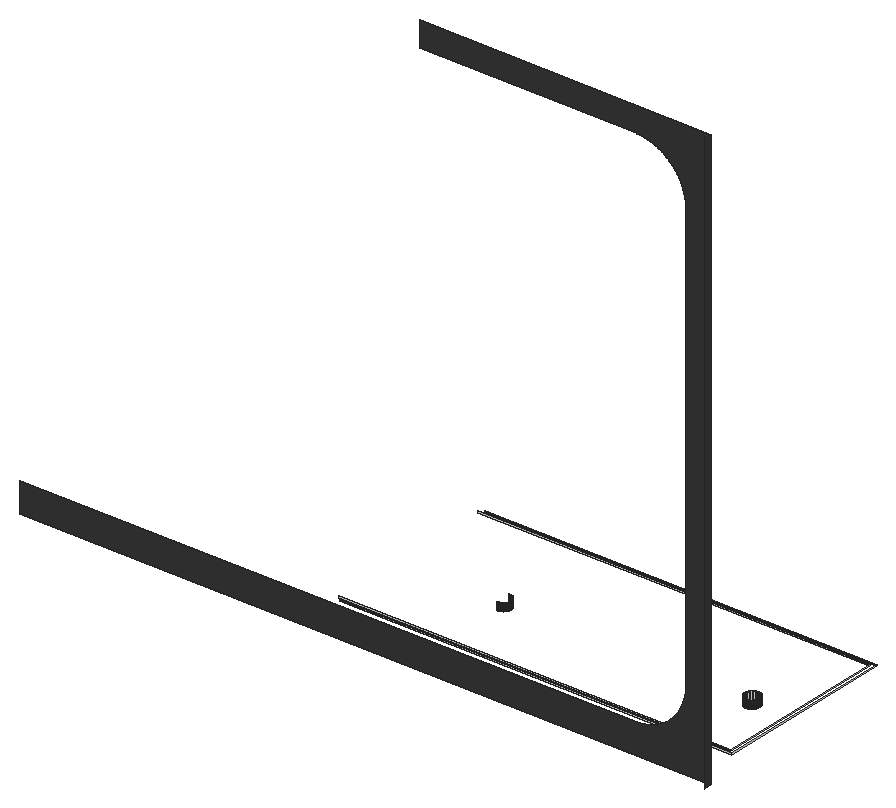
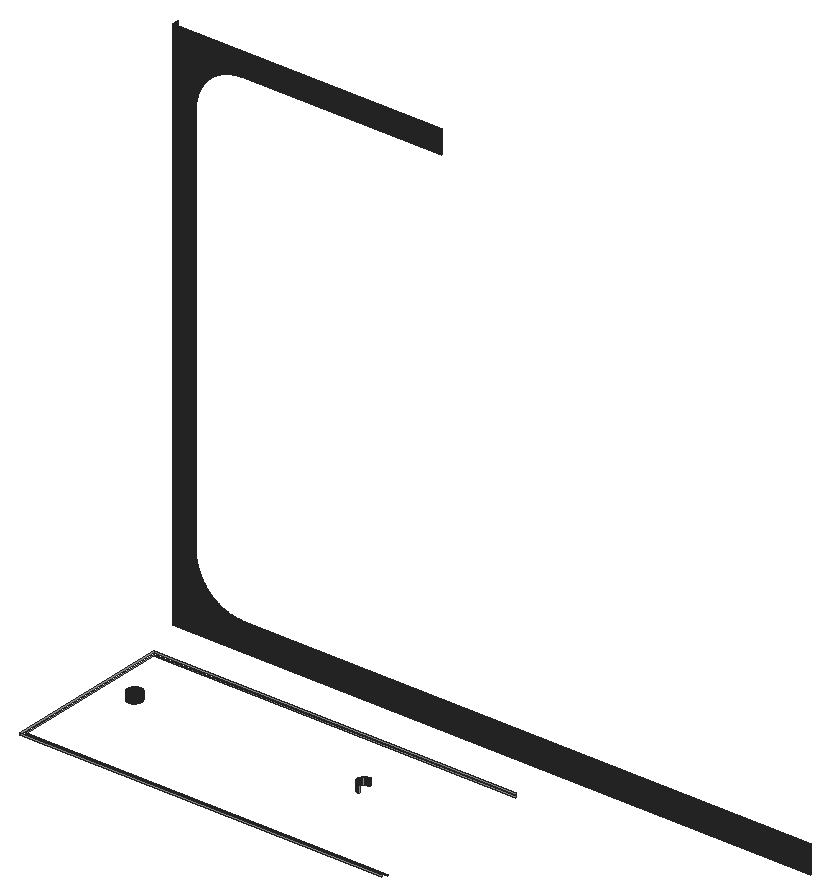
# SketchUp Ruby script. Lengths in inches.
U = 1.inch
M = Sketchup.active_model
def pt(a) = Geom::Point3d.new(a.map { |v| v * U })
def face(e, loops, mat)
  f = e.add_face(loops[0].map { |a| pt(a) })
  loops[1..].each { |l| e.add_face(l.map { |a| pt(a) }).erase! }
  f.material = f.back_material = mat if mat
  f
end
# faces: each face lists its corners as indices into pts; further lists are holes
def faces(e, pts, list, mat = nil) = list.each { |f| face(e, (f[0].is_a?(Array) ? f : [f]).map { |l| l.map { |i| pts[i] } }, mat) }
# xy, xz, yz: faces in a plane at the given z, y or x. An outline is a flat list of corners, or four numbers for a rectangle; further outlines are holes
def ring(l) = l.size == 4 ? [[l[0], l[1]], [l[2], l[1]], [l[2], l[3]], [l[0], l[3]]] : l.each_slice(2).to_a
def flat(e, list, mat, &to3) = list.each { |f| face(e, (f[0].is_a?(Array) ? f : [f]).map { |l| ring(l).map { |u, v| to3.(u, v) } }, mat) }
def xy(e, z, list, mat = nil) = flat(e, list, mat) { |x, y| [x, y, z] }
def xz(e, y, list, mat = nil) = flat(e, list, mat) { |x, z| [x, y, z] }
def yz(e, x, list, mat = nil) = flat(e, list, mat) { |y, z| [x, y, z] }
def lines(e, pts, list) = list.each { |a, b| e.add_line(pt(pts[a]), pt(pts[b])) }
# prism: a flat outline (further loops are holes) pulled along v
def prism(e, loops, v, mat = nil)
  f = face(e, loops, mat); d = Geom::Vector3d.new(v.map { |x| x * U })
  f.pushpull(f.normal.samedirection?(d) ? d.length : -d.length)
end
def box(e, o, s, mat = nil) = prism(e, [[o, [o[0] + s[0], o[1], o[2]], [o[0] + s[0], o[1] + s[1], o[2]], [o[0], o[1] + s[1], o[2]]]], [0, 0, s[2]], mat)
def at(x, y, z, deg = 0) = Geom::Transformation.translation(pt([x, y, z])) * Geom::Transformation.rotation(ORIGIN, Z_AXIS, deg.degrees)
def axes(o, x, y, z) = Geom::Transformation.new([*x, 0, *y, 0, *z, 0, *pt(o).to_a, 1])
def part(name) = M.definitions.add(name)
# library, detail: a bought-in or finely detailed component or shape, given as its bounding box
def library(name, o, s) = part(name).tap { |d| box(d.entities, o, s) }
def detail(e, o, s) = box(e.add_group.entities, o, s)
def put(e, d, t, mat = nil) = e.add_instance(d, t).tap { |i| i.material = mat if mat }
def group(e, t, mat = nil) = e.add_group.tap { |g| g.transformation = t; g.material = mat if mat }.entities
root = M.entities
M.materials.add("1496 AP 8293 CARBON COPY").color = [58, 58, 58]
xz(root,74,[[46,129,321,129,321,361,205,361,205,351,291.26,351,291.52,350.99,291.79,350.98,292.31,350.96,292.57,350.9375,292.83,350.92,293.61,350.83,294.39,350.71,294.64,350.67,294.9,350.62,295.16,350.5625,295.41,350.51,295.67,350.45,295.92,350.38,296.18,350.32,296.68,350.18,297.18,350.02,297.43,349.9375,297.68,349.85,297.92,349.76,298.17,349.67,298.41,349.58,298.65,349.48,299.13,349.27,299.375,349.16,299.61,349.05,299.85,348.9375,300.08,348.82,300.3125,348.7,300.54,348.58,301,348.32,301.23,348.1875,301.45,348.05,302.11,347.63,302.33,347.48,302.54,347.33,302.76,347.18,302.97,347.03,303.18,346.87,303.38,346.71,303.59,346.54,303.99,346.21,304.1875,346.04,304.38,345.86,304.58,345.6875,304.77,345.51,304.96,345.33,305.14,345.14,305.33,344.96,305.51,344.77,305.6875,344.58,305.86,344.38,306.04,344.1875,306.21,343.99,306.54,343.59,306.71,343.38,306.87,343.18,307.03,342.97,307.18,342.76,307.33,342.54,307.48,342.33,307.63,342.11,308.05,341.45,308.1875,341.23,308.32,341,308.58,340.54,308.7,340.3125,308.82,340.08,308.9375,339.85,309.05,339.61,309.16,339.375,309.27,339.13,309.48,338.65,309.58,338.41,309.67,338.17,309.76,337.92,309.85,337.68,309.9375,337.43,310.02,337.18,310.18,336.68,310.32,336.18,310.38,335.92,310.45,335.67,310.51,335.41,310.5625,335.16,310.62,334.9,310.67,334.64,310.71,334.39,310.83,333.61,310.92,332.83,310.9375,332.57,310.96,332.31,310.98,331.79,310.99,331.52,311,331.26,311,160.74,310.99,160.48,310.98,160.21,310.96,159.69,310.9375,159.43,310.92,159.17,310.83,158.39,310.71,157.61,310.67,157.36,310.62,157.1,310.5625,156.84,310.51,156.59,310.45,156.33,310.38,156.08,310.32,155.82,310.18,155.32,310.02,154.82,309.9375,154.57,309.85,154.32,309.76,154.08,309.67,153.83,309.58,153.59,309.48,153.35,309.27,152.87,309.16,152.625,309.05,152.39,308.9375,152.15,308.82,151.92,308.7,151.6875,308.58,151.46,308.32,151,308.1875,150.77,308.05,150.55,307.63,149.89,307.48,149.67,307.33,149.46,307.18,149.24,307.03,149.03,306.87,148.82,306.71,148.62,306.54,148.41,306.21,148.01,306.04,147.8125,305.86,147.62,305.6875,147.42,305.51,147.23,305.33,147.04,305.14,146.86,304.96,146.67,304.77,146.49,304.58,146.3125,304.38,146.14,304.1875,145.96,303.99,145.79,303.59,145.46,303.38,145.29,303.18,145.13,302.97,144.97,302.76,144.82,302.54,144.67,302.33,144.52,302.11,144.37,301.45,143.95,301.23,143.8125,301,143.68,300.54,143.42,300.3125,143.3,300.08,143.18,299.85,143.0625,299.61,142.95,299.375,142.84,299.13,142.73,298.65,142.52,298.41,142.42,298.17,142.33,297.92,142.24,297.68,142.15,297.43,142.0625,297.18,141.98,296.68,141.82,296.18,141.68,295.92,141.62,295.67,141.55,295.41,141.49,295.16,141.4375,294.9,141.38,294.64,141.33,294.39,141.29,293.61,141.17,292.83,141.08,292.57,141.0625,292.31,141.04,291.79,141.02,291.52,141.01,291.26,141,46,141]],"1496 AP 8293 CARBON COPY")
xz(root,93,[[158,129,314,129.5]])
xz(root,94.5,[[156.5,129,312.5,129.5]])
xz(root,119,[[199.84,129,199.92,132],[199.92,129,200,132],[200,129,200.08,132],[200.08,129,200.16,132],[298.84,129,298.92,132],
  [298.92,129,299,132],[299,129,299.08,132],[299.08,129,299.16,132]])
xz(root,125,[[199.84,129,199.92,132],[199.92,129,200,132],[200,129,200.08,132],[200.08,129,200.16,132],[298.84,129,298.92,132],
  [298.92,129,299,132],[299,129,299.08,132],[299.08,129,299.16,132]])
xz(root,163.5,[[156.5,129,312.5,129.5]])
xz(root,165,[[158,129,314,129.5]])
yz(root,203,[[121.84,129,121.92,132],[121.92,129,122,132],[122,129,122.08,132],[122.08,129,122.16,132]])
yz(root,296,[[121.84,129,121.92,132],[121.92,129,122,132],[122,129,122.08,132],[122.08,129,122.16,132]])
yz(root,302,[[121.84,129,121.92,132],[121.92,129,122,132],[122,129,122.08,132],[122.08,129,122.16,132]])
yz(root,312.5,[[94.5,129,163.5,129.5]])
yz(root,314,[[93,129,165,129.5]])
yz(root,321,[[71,129,74,361]],"1496 AP 8293 CARBON COPY")
p = [[199.61,119.03,129],[199.53,119.04,129],[199.53,119.04,132],[199.61,119.03,132],[199.6875,119.02,129],[199.6875,119.02,132],
  [199.76,119.01,129],[199.76,119.01,132],[199.84,119,129],[199.84,119,132],[200.24,119.01,129],[200.16,119,129],
  [200.16,119,132],[200.24,119.01,132],[200.3125,119.02,129],[200.3125,119.02,132],[200.39,119.03,129],[200.39,119.03,132],
  [200.47,119.04,129],[200.47,119.04,132],[200.55,119.05,129],[200.55,119.05,132],[298.53,119.04,129],[298.45,119.05,129],
  [298.45,119.05,132],[298.53,119.04,132],[298.61,119.03,129],[298.61,119.03,132],[298.6875,119.02,129],[298.6875,119.02,132],
  [298.76,119.01,129],[298.76,119.01,132],[298.84,119,129],[298.84,119,132],[299.24,119.01,129],[299.16,119,129],
  [299.16,119,132],[299.24,119.01,132],[299.3125,119.02,129],[299.3125,119.02,132],[299.39,119.03,129],[299.39,119.03,132],
  [299.47,119.04,129],[299.47,119.04,132],[299.55,119.05,129],[299.55,119.05,132],[200.625,119.07,129],[200.625,119.07,132],
  [200.7,119.08,129],[200.7,119.08,132],[200.78,119.1,129],[200.78,119.1,132],[200.85,119.125,129],[200.85,119.125,132],
  [200.93,119.15,129],[200.93,119.15,132],[201,119.17,129],[201,119.17,132],[298.07,119.15,129],[298,119.17,129],
  [298,119.17,132],[298.07,119.15,132],[298.15,119.125,129],[298.15,119.125,132],[298.22,119.1,129],[298.22,119.1,132],
  [298.3,119.08,129],[298.3,119.08,132],[298.375,119.07,129],[298.375,119.07,132],[299.625,119.07,129],[299.625,119.07,132],
  [299.7,119.08,129],[299.7,119.08,132],[299.78,119.1,129],[299.78,119.1,132],[299.85,119.125,129],[299.85,119.125,132],
  [299.93,119.15,129],[299.93,119.15,132],[300,119.17,129],[300,119.17,132],[201.08,119.2,129],[201.08,119.2,132],
  [201.15,119.23,129],[201.15,119.23,132],[201.22,119.26,129],[201.22,119.26,132],[297.85,119.23,129],[297.78,119.26,129],
  [297.78,119.26,132],[297.85,119.23,132],[297.92,119.2,129],[297.92,119.2,132],[300.08,119.2,129],[300.08,119.2,132],
  [300.15,119.23,129],[300.15,119.23,132],[300.22,119.26,129],[300.22,119.26,132],[201.29,119.29,129],[201.29,119.29,132],
  [201.36,119.33,129],[201.36,119.33,132],[201.43,119.36,129],[201.43,119.36,132],[297.64,119.33,129],[297.57,119.36,129],
  [297.57,119.36,132],[297.64,119.33,132],[297.71,119.29,129],[297.71,119.29,132],[300.29,119.29,129],[300.29,119.29,132],
  [300.36,119.33,129],[300.36,119.33,132],[300.43,119.36,129],[300.43,119.36,132],[201.5,119.4,129],[201.5,119.4,132],
  [201.57,119.44,129],[201.57,119.44,132],[201.63,119.48,129],[201.63,119.48,132],[297.43,119.44,129],[297.37,119.48,129],
  [297.37,119.48,132],[297.43,119.44,132],[297.5,119.4,129],[297.5,119.4,132],[300.5,119.4,129],[300.5,119.4,132],
  [300.57,119.44,129],[300.57,119.44,132],[300.63,119.48,129],[300.63,119.48,132],[201.7,119.53,129],[201.7,119.53,132],
  [201.76,119.57,129],[201.76,119.57,132],[297.3,119.53,129],[297.24,119.57,129],[297.24,119.57,132],[297.3,119.53,132],
  [300.7,119.53,129],[300.7,119.53,132],[300.76,119.57,129],[300.76,119.57,132],[201.83,119.62,129],[201.83,119.62,132],
  [201.89,119.67,129],[201.89,119.67,132],[297.17,119.62,129],[297.11,119.67,129],[297.11,119.67,132],[297.17,119.62,132],
  [300.83,119.62,129],[300.83,119.62,132],[300.89,119.67,129],[300.89,119.67,132],[201.95,119.72,129],[201.95,119.72,132],
  [202.01,119.77,129],[202.01,119.77,132],[297.05,119.72,129],[296.99,119.77,129],[296.99,119.77,132],[297.05,119.72,132],
  [300.95,119.72,129],[300.95,119.72,132],[301.01,119.77,129],[301.01,119.77,132],[202.07,119.82,129],[202.07,119.82,132],
  [202.12,119.88,129],[202.12,119.88,132],[296.93,119.82,129],[296.88,119.88,129],[296.88,119.88,132],[296.93,119.82,132],
  [301.07,119.82,129],[301.07,119.82,132],[301.12,119.88,129],[301.12,119.88,132],[202.18,119.93,129],[202.18,119.93,132],
  [202.23,119.99,129],[202.23,119.99,132],[296.82,119.93,129],[296.77,119.99,129],[296.77,119.99,132],[296.82,119.93,132],
  [301.18,119.93,129],[301.18,119.93,132],[301.23,119.99,129],[301.23,119.99,132],[202.28,120.05,129],[202.28,120.05,132],
  [296.72,120.05,129],[296.72,120.05,132],[301.28,120.05,129],[301.28,120.05,132],[202.33,120.11,129],[202.33,120.11,132],
  [202.38,120.17,129],[202.38,120.17,132],[296.67,120.11,129],[296.62,120.17,129],[296.62,120.17,132],[296.67,120.11,132],
  [301.33,120.11,129],[301.33,120.11,132],[301.38,120.17,129],[301.38,120.17,132],[202.43,120.24,129],[202.43,120.24,132],
  [202.47,120.3,129],[202.47,120.3,132],[296.57,120.24,129],[296.53,120.3,129],[296.53,120.3,132],[296.57,120.24,132],
  [301.43,120.24,129],[301.43,120.24,132],[301.47,120.3,129],[301.47,120.3,132],[202.52,120.37,129],[202.52,120.37,132],
  [296.48,120.37,129],[296.48,120.37,132],[301.52,120.37,129],[301.52,120.37,132],[202.56,120.43,129],[202.56,120.43,132],
  [202.6,120.5,129],[202.6,120.5,132],[296.44,120.43,129],[296.4,120.5,129],[296.4,120.5,132],[296.44,120.43,132],
  [301.56,120.43,129],[301.56,120.43,132],[301.6,120.5,129],[301.6,120.5,132],[202.64,120.57,129],[202.64,120.57,132],
  [296.36,120.57,129],[296.36,120.57,132],[301.64,120.57,129],[301.64,120.57,132],[202.67,120.64,129],[202.67,120.64,132],
  [202.71,120.71,129],[202.71,120.71,132],[296.33,120.64,129],[296.29,120.71,129],[296.29,120.71,132],[296.33,120.64,132],
  [301.67,120.64,129],[301.67,120.64,132],[301.71,120.71,129],[301.71,120.71,132],[202.74,120.78,129],[202.74,120.78,132],
  [296.26,120.78,129],[296.26,120.78,132],[301.74,120.78,129],[301.74,120.78,132],[202.77,120.85,129],[202.77,120.85,132],
  [296.23,120.85,129],[296.23,120.85,132],[301.77,120.85,129],[301.77,120.85,132],[202.8,120.92,129],[202.8,120.92,132],
  [202.83,121,129],[202.83,121,132],[296.2,120.92,129],[296.17,121,129],[296.17,121,132],[296.2,120.92,132],
  [301.8,120.92,129],[301.8,120.92,132],[301.83,121,129],[301.83,121,132],[202.85,121.07,129],[202.85,121.07,132],
  [296.15,121.07,129],[296.15,121.07,132],[301.85,121.07,129],[301.85,121.07,132],[202.875,121.15,129],[202.875,121.15,132],
  [202.9,121.22,129],[202.9,121.22,132],[296.125,121.15,129],[296.1,121.22,129],[296.1,121.22,132],[296.125,121.15,132],
  [301.875,121.15,129],[301.875,121.15,132],[301.9,121.22,129],[301.9,121.22,132],[202.92,121.3,129],[202.92,121.3,132],
  [296.08,121.3,129],[296.08,121.3,132],[301.92,121.3,129],[301.92,121.3,132],[202.93,121.375,129],[202.93,121.375,132],
  [296.07,121.375,129],[296.07,121.375,132],[301.93,121.375,129],[301.93,121.375,132],[202.95,121.45,129],[202.95,121.45,132],
  [296.05,121.45,129],[296.05,121.45,132],[301.95,121.45,129],[301.95,121.45,132],[202.96,121.53,129],[202.96,121.53,132],
  [202.97,121.61,129],[202.97,121.61,132],[296.04,121.53,129],[296.03,121.61,129],[296.03,121.61,132],[296.04,121.53,132],
  [301.96,121.53,129],[301.96,121.53,132],[301.97,121.61,129],[301.97,121.61,132],[202.98,121.6875,129],[202.98,121.6875,132],
  [296.02,121.6875,129],[296.02,121.6875,132],[301.98,121.6875,129],[301.98,121.6875,132],[202.99,121.76,129],[202.99,121.76,132],
  [296.01,121.76,129],[296.01,121.76,132],[301.99,121.76,129],[301.99,121.76,132],[203,121.84,129],[203,121.84,132],
  [296,121.84,129],[296,121.84,132],[302,121.84,129],[302,121.84,132],[202.98,122.3125,129],[202.99,122.24,129],
  [202.99,122.24,132],[202.98,122.3125,132],[203,122.16,129],[203,122.16,132],[296,122.16,129],[296.01,122.24,129],
  [296.01,122.24,132],[296,122.16,132],[296.02,122.3125,129],[296.02,122.3125,132],[301.98,122.3125,129],[301.99,122.24,129],
  [301.99,122.24,132],[301.98,122.3125,132],[302,122.16,129],[302,122.16,132],[202.97,122.39,129],[202.97,122.39,132],
  [296.03,122.39,129],[296.03,122.39,132],[301.97,122.39,129],[301.97,122.39,132],[202.96,122.47,129],[202.96,122.47,132],
  [296.04,122.47,129],[296.04,122.47,132],[301.96,122.47,129],[301.96,122.47,132],[202.93,122.625,129],[202.95,122.55,129],
  [202.95,122.55,132],[202.93,122.625,132],[296.05,122.55,129],[296.05,122.55,132],[296.07,122.625,129],[296.07,122.625,132],
  [301.93,122.625,129],[301.95,122.55,129],[301.95,122.55,132],[301.93,122.625,132],[202.92,122.7,129],[202.92,122.7,132],
  [296.08,122.7,129],[296.08,122.7,132],[301.92,122.7,129],[301.92,122.7,132],[202.9,122.78,129],[202.9,122.78,132],
  [296.1,122.78,129],[296.1,122.78,132],[301.9,122.78,129],[301.9,122.78,132],[202.875,122.85,129],[202.875,122.85,132],
  [296.125,122.85,129],[296.125,122.85,132],[301.875,122.85,129],[301.875,122.85,132],[202.83,123,129],[202.85,122.93,129],
  [202.85,122.93,132],[202.83,123,132],[296.15,122.93,129],[296.15,122.93,132],[296.17,123,129],[296.17,123,132],
  [301.83,123,129],[301.85,122.93,129],[301.85,122.93,132],[301.83,123,132],[202.8,123.08,129],[202.8,123.08,132],
  [296.2,123.08,129],[296.2,123.08,132],[301.8,123.08,129],[301.8,123.08,132],[202.74,123.22,129],[202.77,123.15,129],
  [202.77,123.15,132],[202.74,123.22,132],[296.23,123.15,129],[296.23,123.15,132],[296.26,123.22,129],[296.26,123.22,132],
  [301.74,123.22,129],[301.77,123.15,129],[301.77,123.15,132],[301.74,123.22,132],[202.71,123.29,129],[202.71,123.29,132],
  [296.29,123.29,129],[296.29,123.29,132],[301.71,123.29,129],[301.71,123.29,132],[202.67,123.36,129],[202.67,123.36,132],
  [296.33,123.36,129],[296.33,123.36,132],[301.67,123.36,129],[301.67,123.36,132],[202.6,123.5,129],[202.64,123.43,129],
  [202.64,123.43,132],[202.6,123.5,132],[296.36,123.43,129],[296.36,123.43,132],[296.4,123.5,129],[296.4,123.5,132],
  [301.6,123.5,129],[301.64,123.43,129],[301.64,123.43,132],[301.6,123.5,132],[202.56,123.57,129],[202.56,123.57,132],
  [296.44,123.57,129],[296.44,123.57,132],[301.56,123.57,129],[301.56,123.57,132],[202.47,123.7,129],[202.52,123.63,129],
  [202.52,123.63,132],[202.47,123.7,132],[296.48,123.63,129],[296.48,123.63,132],[296.53,123.7,129],[296.53,123.7,132],
  [301.47,123.7,129],[301.52,123.63,129],[301.52,123.63,132],[301.47,123.7,132],[202.43,123.76,129],[202.43,123.76,132],
  [296.57,123.76,129],[296.57,123.76,132],[301.43,123.76,129],[301.43,123.76,132],[202.33,123.89,129],[202.38,123.83,129],
  [202.38,123.83,132],[202.33,123.89,132],[296.62,123.83,129],[296.62,123.83,132],[296.67,123.89,129],[296.67,123.89,132],
  [301.33,123.89,129],[301.38,123.83,129],[301.38,123.83,132],[301.33,123.89,132],[202.23,124.01,129],[202.28,123.95,129],
  [202.28,123.95,132],[202.23,124.01,132],[296.72,123.95,129],[296.72,123.95,132],[296.77,124.01,129],[296.77,124.01,132],
  [301.23,124.01,129],[301.28,123.95,129],[301.28,123.95,132],[301.23,124.01,132],[202.18,124.07,129],[202.18,124.07,132],
  [296.82,124.07,129],[296.82,124.07,132],[301.18,124.07,129],[301.18,124.07,132],[202.07,124.18,129],[202.12,124.12,129],
  [202.12,124.12,132],[202.07,124.18,132],[296.88,124.12,129],[296.88,124.12,132],[296.93,124.18,129],[296.93,124.18,132],
  [301.07,124.18,129],[301.12,124.12,129],[301.12,124.12,132],[301.07,124.18,132],[201.95,124.28,129],[202.01,124.23,129],
  [202.01,124.23,132],[201.95,124.28,132],[296.99,124.23,129],[296.99,124.23,132],[297.05,124.28,129],[297.05,124.28,132],
  [300.95,124.28,129],[301.01,124.23,129],[301.01,124.23,132],[300.95,124.28,132],[201.83,124.38,129],[201.89,124.33,129],
  [201.89,124.33,132],[201.83,124.38,132],[297.11,124.33,129],[297.11,124.33,132],[297.17,124.38,129],[297.17,124.38,132],
  [300.83,124.38,129],[300.89,124.33,129],[300.89,124.33,132],[300.83,124.38,132],[201.7,124.47,129],[201.76,124.43,129],
  [201.76,124.43,132],[201.7,124.47,132],[297.24,124.43,129],[297.24,124.43,132],[297.3,124.47,129],[297.3,124.47,132],
  [300.7,124.47,129],[300.76,124.43,129],[300.76,124.43,132],[300.7,124.47,132],[201.57,124.56,129],[201.63,124.52,129],
  [201.63,124.52,132],[201.57,124.56,132],[297.37,124.52,129],[297.37,124.52,132],[297.43,124.56,129],[297.43,124.56,132],
  [300.57,124.56,129],[300.63,124.52,129],[300.63,124.52,132],[300.57,124.56,132],[201.36,124.67,129],[201.43,124.64,129],
  [201.43,124.64,132],[201.36,124.67,132],[201.5,124.6,129],[201.5,124.6,132],[297.5,124.6,129],[297.5,124.6,132],
  [297.57,124.64,129],[297.57,124.64,132],[297.64,124.67,129],[297.64,124.67,132],[300.36,124.67,129],[300.43,124.64,129],
  [300.43,124.64,132],[300.36,124.67,132],[300.5,124.6,129],[300.5,124.6,132],[201.15,124.77,129],[201.22,124.74,129],
  [201.22,124.74,132],[201.15,124.77,132],[201.29,124.71,129],[201.29,124.71,132],[297.71,124.71,129],[297.71,124.71,132],
  [297.78,124.74,129],[297.78,124.74,132],[297.85,124.77,129],[297.85,124.77,132],[300.15,124.77,129],[300.22,124.74,129],
  [300.22,124.74,132],[300.15,124.77,132],[300.29,124.71,129],[300.29,124.71,132],[200.93,124.85,129],[201,124.83,129],
  [201,124.83,132],[200.93,124.85,132],[201.08,124.8,129],[201.08,124.8,132],[297.92,124.8,129],[297.92,124.8,132],
  [298,124.83,129],[298,124.83,132],[298.07,124.85,129],[298.07,124.85,132],[299.93,124.85,129],[300,124.83,129],
  [300,124.83,132],[299.93,124.85,132],[300.08,124.8,129],[300.08,124.8,132],[200.47,124.96,129],[200.55,124.95,129],
  [200.55,124.95,132],[200.47,124.96,132],[200.625,124.93,129],[200.625,124.93,132],[200.7,124.92,129],[200.7,124.92,132],
  [200.78,124.9,129],[200.78,124.9,132],[200.85,124.875,129],[200.85,124.875,132],[298.15,124.875,129],[298.15,124.875,132],
  [298.22,124.9,129],[298.22,124.9,132],[298.3,124.92,129],[298.3,124.92,132],[298.375,124.93,129],[298.375,124.93,132],
  [298.45,124.95,129],[298.45,124.95,132],[298.53,124.96,129],[298.53,124.96,132],[299.47,124.96,129],[299.55,124.95,129],
  [299.55,124.95,132],[299.47,124.96,132],[299.625,124.93,129],[299.625,124.93,132],[299.7,124.92,129],[299.7,124.92,132],
  [299.78,124.9,129],[299.78,124.9,132],[299.85,124.875,129],[299.85,124.875,132],[199.61,124.97,129],[199.6875,124.98,129],
  [199.6875,124.98,132],[199.61,124.97,132],[199.76,124.99,129],[199.76,124.99,132],[199.84,125,129],[199.84,125,132],
  [200.16,125,129],[200.24,124.99,129],[200.24,124.99,132],[200.16,125,132],[200.3125,124.98,129],[200.3125,124.98,132],
  [200.39,124.97,129],[200.39,124.97,132],[298.61,124.97,129],[298.61,124.97,132],[298.6875,124.98,129],[298.6875,124.98,132],
  [298.76,124.99,129],[298.76,124.99,132],[298.84,125,129],[298.84,125,132],[299.16,125,129],[299.24,124.99,129],
  [299.24,124.99,132],[299.16,125,132],[299.3125,124.98,129],[299.3125,124.98,132],[299.39,124.97,129],[299.39,124.97,132]]
faces(root,p,[[0,1,2,3],[4,0,3,5],[6,4,5,7],[8,6,7,9],[10,11,12,13],[14,10,13,15],[16,14,15,17],[18,16,17,19],
  [20,18,19,21],[22,23,24,25],[26,22,25,27],[28,26,27,29],[30,28,29,31],[32,30,31,33],[34,35,36,37],[38,34,37,39],
  [40,38,39,41],[42,40,41,43],[44,42,43,45],[46,20,21,47],[48,46,47,49],[50,48,49,51],[52,50,51,53],[54,52,53,55],
  [56,54,55,57],[58,59,60,61],[62,58,61,63],[64,62,63,65],[66,64,65,67],[68,66,67,69],[23,68,69,24],[70,44,45,71],
  [72,70,71,73],[74,72,73,75],[76,74,75,77],[78,76,77,79],[80,78,79,81],[82,56,57,83],[84,82,83,85],[86,84,85,87],
  [88,89,90,91],[92,88,91,93],[59,92,93,60],[94,80,81,95],[96,94,95,97],[98,96,97,99],[100,86,87,101],[102,100,101,103],
  [104,102,103,105],[106,107,108,109],[110,106,109,111],[89,110,111,90],[112,98,99,113],[114,112,113,115],[116,114,115,117],[118,104,105,119],
  [120,118,119,121],[122,120,121,123],[124,125,126,127],[128,124,127,129],[107,128,129,108],[130,116,117,131],[132,130,131,133],[134,132,133,135],
  [136,122,123,137],[138,136,137,139],[140,141,142,143],[125,140,143,126],[144,134,135,145],[146,144,145,147],[148,138,139,149],[150,148,149,151],
  [152,153,154,155],[141,152,155,142],[156,146,147,157],[158,156,157,159],[160,150,151,161],[162,160,161,163],[164,165,166,167],[153,164,167,154],
  [168,158,159,169],[170,168,169,171],[172,162,163,173],[174,172,173,175],[176,177,178,179],[165,176,179,166],[180,170,171,181],[182,180,181,183],
  [184,174,175,185],[186,184,185,187],[188,189,190,191],[177,188,191,178],[192,182,183,193],[194,192,193,195],[196,186,187,197],[189,198,199,190],
  [200,194,195,201],[202,196,197,203],[204,202,203,205],[206,207,208,209],[198,206,209,199],[210,200,201,211],[212,210,211,213],[214,204,205,215],
  [216,214,215,217],[218,219,220,221],[207,218,221,208],[222,212,213,223],[224,222,223,225],[226,216,217,227],[219,228,229,220],[230,224,225,231],
  [232,226,227,233],[234,232,233,235],[236,237,238,239],[228,236,239,229],[240,230,231,241],[242,240,241,243],[244,234,235,245],[237,246,247,238],
  [248,242,243,249],[250,244,245,251],[252,250,251,253],[254,255,256,257],[246,254,257,247],[258,248,249,259],[260,258,259,261],[262,252,253,263],
  [255,264,265,256],[266,260,261,267],[268,262,263,269],[264,270,271,265],[272,266,267,273],[274,268,269,275],[276,274,275,277],[278,279,280,281],
  [270,278,281,271],[282,272,273,283],[284,282,283,285],[286,276,277,287],[279,288,289,280],[290,284,285,291],[292,286,287,293],[294,292,293,295],
  [296,297,298,299],[288,296,299,289],[300,290,291,301],[302,300,301,303],[304,294,295,305],[297,306,307,298],[308,302,303,309],[310,304,305,311],
  [306,312,313,307],[314,308,309,315],[316,310,311,317],[312,318,319,313],[320,314,315,321],[322,316,317,323],[324,322,323,325],[326,327,328,329],
  [318,326,329,319],[330,320,321,331],[332,330,331,333],[334,324,325,335],[327,336,337,328],[338,332,333,339],[340,334,335,341],[336,342,343,337],
  [344,338,339,345],[346,340,341,347],[342,348,349,343],[350,344,345,351],[352,353,354,355],[353,356,357,354],[358,359,360,361],[359,362,363,360],
  [364,365,366,367],[365,368,369,366],[370,352,355,371],[362,372,373,363],[374,364,367,375],[376,370,371,377],[372,378,379,373],[380,374,375,381],
  [382,383,384,385],[383,376,377,384],[378,386,387,379],[386,388,389,387],[390,391,392,393],[391,380,381,392],[394,382,385,395],[388,396,397,389],
  [398,390,393,399],[400,394,395,401],[396,402,403,397],[404,398,399,405],[406,400,401,407],[402,408,409,403],[410,404,405,411],[412,413,414,415],
  [413,406,407,414],[408,416,417,409],[416,418,419,417],[420,421,422,423],[421,410,411,422],[424,412,415,425],[418,426,427,419],[428,420,423,429],
  [430,431,432,433],[431,424,425,432],[426,434,435,427],[434,436,437,435],[438,439,440,441],[439,428,429,440],[442,430,433,443],[436,444,445,437],
  [446,438,441,447],[448,442,443,449],[444,450,451,445],[452,446,447,453],[454,455,456,457],[455,448,449,456],[450,458,459,451],[458,460,461,459],
  [462,463,464,465],[463,452,453,464],[466,454,457,467],[460,468,469,461],[470,462,465,471],[472,473,474,475],[473,466,467,474],[468,476,477,469],
  [476,478,479,477],[480,481,482,483],[481,470,471,482],[484,472,475,485],[478,486,487,479],[488,480,483,489],[490,491,492,493],[491,484,485,492],
  [486,494,495,487],[494,496,497,495],[498,499,500,501],[499,488,489,500],[502,503,504,505],[503,490,493,504],[496,506,507,497],[506,508,509,507],
  [510,511,512,513],[511,498,501,512],[514,502,505,515],[508,516,517,509],[518,510,513,519],[520,521,522,523],[521,514,515,522],[516,524,525,517],
  [524,526,527,525],[528,529,530,531],[529,518,519,530],[532,533,534,535],[533,520,523,534],[526,536,537,527],[536,538,539,537],[540,541,542,543],
  [541,528,531,542],[544,545,546,547],[545,532,535,546],[538,548,549,539],[548,550,551,549],[552,553,554,555],[553,540,543,554],[556,557,558,559],
  [557,544,547,558],[550,560,561,551],[560,562,563,561],[564,565,566,567],[565,552,555,566],[568,569,570,571],[569,556,559,570],[562,572,573,563],
  [572,574,575,573],[576,577,578,579],[577,564,567,578],[580,581,582,583],[581,584,585,582],[584,568,571,585],[574,586,587,575],[586,588,589,587],
  [588,590,591,589],[592,593,594,595],[593,596,597,594],[596,576,579,597],[598,599,600,601],[599,602,603,600],[602,580,583,603],[590,604,605,591],
  [604,606,607,605],[606,608,609,607],[610,611,612,613],[611,614,615,612],[614,592,595,615],[616,617,618,619],[617,620,621,618],[620,598,601,621],
  [608,622,623,609],[622,624,625,623],[624,626,627,625],[628,629,630,631],[629,632,633,630],[632,610,613,633],[634,635,636,637],[635,638,639,636],
  [638,640,641,639],[640,642,643,641],[642,644,645,643],[644,616,619,645],[626,646,647,627],[646,648,649,647],[648,650,651,649],[650,652,653,651],
  [652,654,655,653],[654,656,657,655],[658,659,660,661],[659,662,663,660],[662,664,665,663],[664,666,667,665],[666,668,669,667],[668,628,631,669],
  [670,671,672,673],[671,674,675,672],[674,676,677,675],[678,679,680,681],[679,682,683,680],[682,684,685,683],[684,634,637,685],[656,686,687,657],
  [686,688,689,687],[688,690,691,689],[690,692,693,691],[694,695,696,697],[695,698,699,696],[698,700,701,699],[700,658,661,701]])
